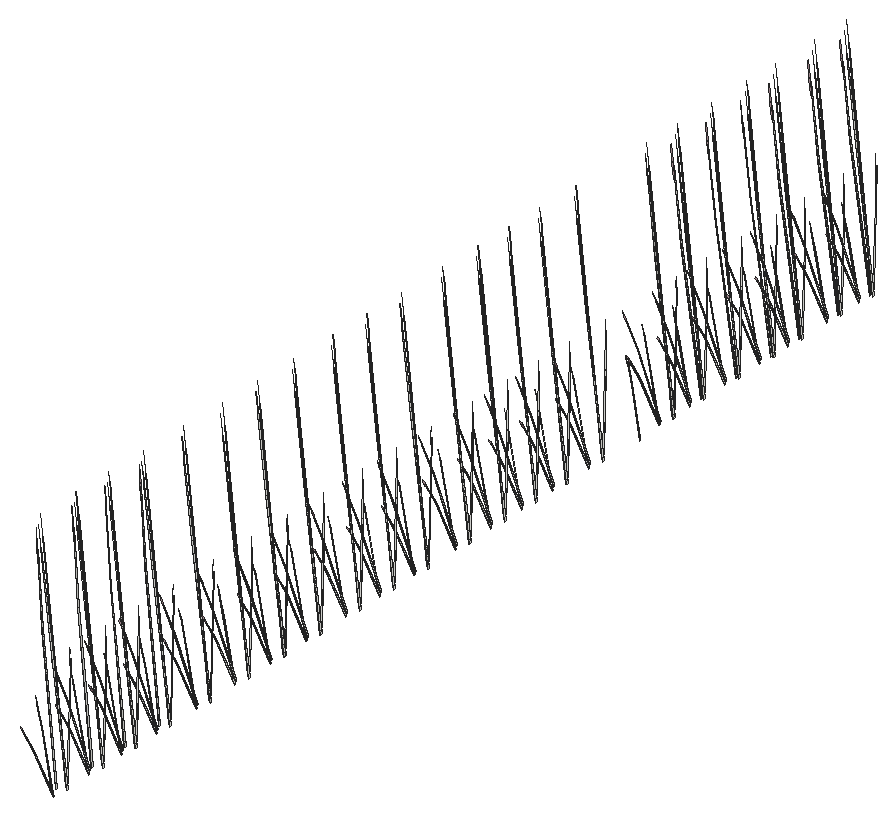
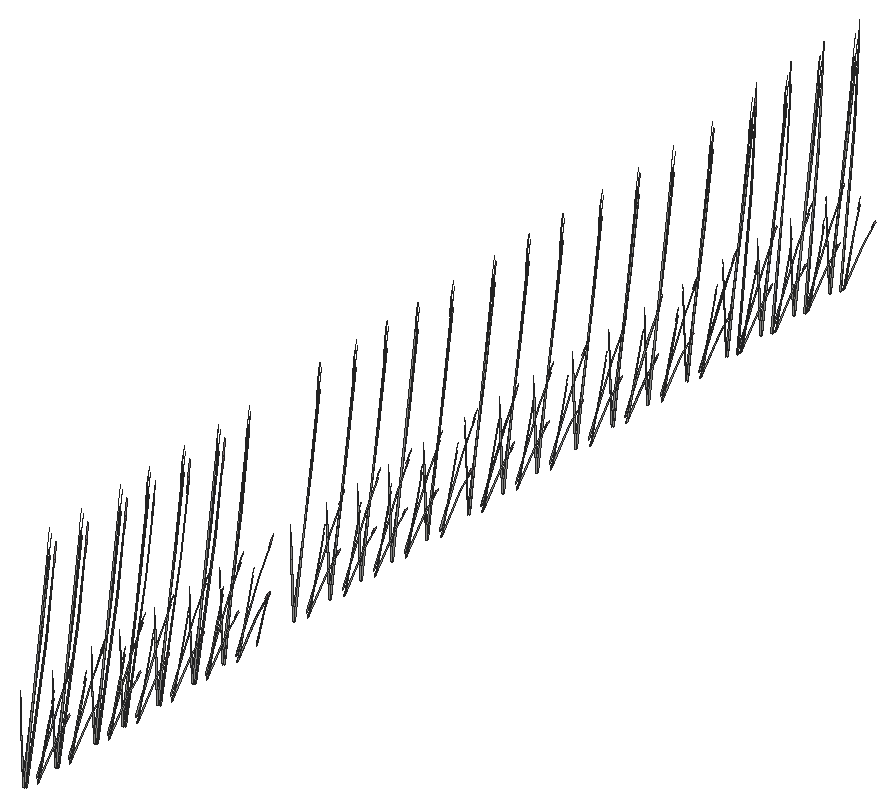
# SketchUp Ruby script. Lengths in inches.
U = 1.inch
M = Sketchup.active_model
def pt(a) = Geom::Point3d.new(a.map { |v| v * U })
def face(e, loops, mat)
  f = e.add_face(loops[0].map { |a| pt(a) })
  loops[1..].each { |l| e.add_face(l.map { |a| pt(a) }).erase! }
  f.material = f.back_material = mat if mat
  f
end
# faces: each face lists its corners as indices into pts; further lists are holes
def faces(e, pts, list, mat = nil) = list.each { |f| face(e, (f[0].is_a?(Array) ? f : [f]).map { |l| l.map { |i| pts[i] } }, mat) }
# xy, xz, yz: faces in a plane at the given z, y or x. An outline is a flat list of corners, or four numbers for a rectangle; further outlines are holes
def ring(l) = l.size == 4 ? [[l[0], l[1]], [l[2], l[1]], [l[2], l[3]], [l[0], l[3]]] : l.each_slice(2).to_a
def flat(e, list, mat, &to3) = list.each { |f| face(e, (f[0].is_a?(Array) ? f : [f]).map { |l| ring(l).map { |u, v| to3.(u, v) } }, mat) }
def xy(e, z, list, mat = nil) = flat(e, list, mat) { |x, y| [x, y, z] }
def xz(e, y, list, mat = nil) = flat(e, list, mat) { |x, z| [x, y, z] }
def yz(e, x, list, mat = nil) = flat(e, list, mat) { |y, z| [x, y, z] }
def lines(e, pts, list) = list.each { |a, b| e.add_line(pt(pts[a]), pt(pts[b])) }
# prism: a flat outline (further loops are holes) pulled along v
def prism(e, loops, v, mat = nil)
  f = face(e, loops, mat); d = Geom::Vector3d.new(v.map { |x| x * U })
  f.pushpull(f.normal.samedirection?(d) ? d.length : -d.length)
end
def box(e, o, s, mat = nil) = prism(e, [[o, [o[0] + s[0], o[1], o[2]], [o[0] + s[0], o[1] + s[1], o[2]], [o[0], o[1] + s[1], o[2]]]], [0, 0, s[2]], mat)
def at(x, y, z, deg = 0) = Geom::Transformation.translation(pt([x, y, z])) * Geom::Transformation.rotation(ORIGIN, Z_AXIS, deg.degrees)
def axes(o, x, y, z) = Geom::Transformation.new([*x, 0, *y, 0, *z, 0, *pt(o).to_a, 1])
def part(name) = M.definitions.add(name)
# library, detail: a bought-in or finely detailed component or shape, given as its bounding box
def library(name, o, s) = part(name).tap { |d| box(d.entities, o, s) }
def detail(e, o, s) = box(e.add_group.entities, o, s)
def put(e, d, t, mat = nil) = e.add_instance(d, t).tap { |i| i.material = mat if mat }
def group(e, t, mat = nil) = e.add_group.tap { |g| g.transformation = t; g.material = mat if mat }.entities
root = M.entities
M.materials.add("LightPink_Translucent").color = [144, 107, 117]
M.materials["LightPink_Translucent"].alpha = 0.75
c1 = part("blade")
p = [[2.15,0.21,22],[0,0.17,0],[0.09,0.45,0],[2.18,0.31,22],[2.29,0.31,22],[0.38,0.45,0],
  [2.48,0.24,33],[2.49,0.24,33],[2.48,0.22,33]]
faces(c1.entities,p,[[0,1,2,3],[4,5,2,3],[6,3,4,7],[8,0,3,6]])
c2 = part("seeds")
p = [[0.3,-0.1,1.38],[-0.01,-0.03,1.59],[-0.01,-0.03,0.03],[0.14,-0.07,-0.07],[0.29,-0.03,3],[0.15,0.01,3.11]]
faces(c2.entities,p,[[0,1,2,3],[1,0,4,5]],"LightPink_Translucent")
c3 = part("blade with seeds")
put(c3.entities,c1,at(0,0,0))
put(c3.entities,c2,axes([2.4,0.25,30.99],[1.5799,-0.05474,1.17369],[-0.12525,1.92788,0.29478],[-0.07173,-0.02425,1.56792]))
put(root,c3,axes([332.39,452.5,49.78],[-0.47255,-0.19538,-0.43871],[0.28245,-0.35034,0],[-0.10763,-0.0445,1.3917]))
put(root,c3,axes([332.39,462.02,49.78],[-0.47255,-0.19538,-0.43871],[0.28245,-0.35034,0],[-0.10763,-0.0445,1.3917]))
put(root,c3,axes([332.39,471.57,49.78],[-0.47255,-0.19538,-0.43871],[0.28245,-0.35034,0],[-0.10763,-0.0445,1.3917]))
put(root,c3,axes([332.39,479.37,49.78],[-0.47255,-0.19538,-0.43871],[0.28245,-0.35034,0],[-0.10763,-0.0445,1.3917]))
put(root,c3,axes([332.39,490.07,49.78],[-0.47255,-0.19538,-0.43871],[0.28245,-0.35034,0],[-0.10763,-0.0445,1.3917]))
put(root,c3,axes([332.39,498.85,49.78],[-0.47255,-0.19538,-0.43871],[0.28245,-0.35034,0],[-0.10763,-0.0445,1.3917]))
put(root,c3,axes([332.18,275.01,49.32],[-0.04891,0.05148,1.55816],[-0.49427,0.11098,-0.23804],[-0.1194,-0.10096,0.26541]))
put(root,c3,axes([332.18,284.8125,49.32],[-0.04891,0.05148,1.55816],[-0.49427,0.11098,-0.23804],[-0.1194,-0.10096,0.26541]))
put(root,c3,axes([332.18,293.79,49.32],[-0.04891,0.05148,1.55816],[-0.49427,0.11098,-0.23804],[-0.1194,-0.10096,0.26541]))
put(root,c3,axes([332.18,303.27,49.32],[-0.04891,0.05148,1.55816],[-0.49427,0.11098,-0.23804],[-0.1194,-0.10096,0.26541]))
put(root,c3,axes([332.18,314.26,49.32],[-0.04891,0.05148,1.55816],[-0.49427,0.11098,-0.23804],[-0.1194,-0.10096,0.26541]))
put(root,c3,axes([332.18,324.86,49.32],[-0.04891,0.05148,1.55816],[-0.49427,0.11098,-0.23804],[-0.1194,-0.10096,0.26541]))
put(root,c3,axes([332.18,334.5625,49.32],[-0.04891,0.05148,1.55816],[-0.49427,0.11098,-0.23804],[-0.1194,-0.10096,0.26541]))
put(root,c3,axes([332.18,344.5,49.32],[-0.04891,0.05148,1.55816],[-0.49427,0.11098,-0.23804],[-0.1194,-0.10096,0.26541]))
put(root,c3,axes([332.18,355.22,49.32],[-0.04891,0.05148,1.55816],[-0.49427,0.11098,-0.23804],[-0.1194,-0.10096,0.26541]))
put(root,c3,axes([332.18,364.55,49.32],[-0.04891,0.05148,1.55816],[-0.49427,0.11098,-0.23804],[-0.1194,-0.10096,0.26541]))
put(root,c3,axes([332.18,374.02,49.32],[-0.04891,0.05148,1.55816],[-0.49427,0.11098,-0.23804],[-0.1194,-0.10096,0.26541]))
put(root,c3,axes([332.18,385.33,49.32],[-0.04891,0.05148,1.55816],[-0.49427,0.11098,-0.23804],[-0.1194,-0.10096,0.26541]))
put(root,c3,axes([332.18,395.01,49.32],[-0.04891,0.05148,1.55816],[-0.49427,0.11098,-0.23804],[-0.1194,-0.10096,0.26541]))
put(root,c3,axes([332.18,403.47,49.32],[-0.04891,0.05148,1.55816],[-0.49427,0.11098,-0.23804],[-0.1194,-0.10096,0.26541]))
put(root,c3,axes([332.18,411.9375,49.32],[-0.04891,0.05148,1.55816],[-0.49427,0.11098,-0.23804],[-0.1194,-0.10096,0.26541]))
put(root,c3,axes([332.18,421.83,49.32],[-0.04891,0.05148,1.55816],[-0.49427,0.11098,-0.23804],[-0.1194,-0.10096,0.26541]))
put(root,c3,axes([332.18,441.22,49.32],[-0.04891,0.05148,1.55816],[-0.49427,0.11098,-0.23804],[-0.1194,-0.10096,0.26541]))
put(root,c3,axes([332.18,449.59,49.32],[-0.04891,0.05148,1.55816],[-0.49427,0.11098,-0.23804],[-0.1194,-0.10096,0.26541]))
put(root,c3,axes([332.18,459.11,49.32],[-0.04891,0.05148,1.55816],[-0.49427,0.11098,-0.23804],[-0.1194,-0.10096,0.26541]))
put(root,c3,axes([332.18,468.66,49.32],[-0.04891,0.05148,1.55816],[-0.49427,0.11098,-0.23804],[-0.1194,-0.10096,0.26541]))
put(root,c3,axes([332.18,476.46,49.32],[-0.04891,0.05148,1.55816],[-0.49427,0.11098,-0.23804],[-0.1194,-0.10096,0.26541]))
put(root,c3,axes([332.18,487.16,49.32],[-0.04891,0.05148,1.55816],[-0.49427,0.11098,-0.23804],[-0.1194,-0.10096,0.26541]))
put(root,c3,axes([332.18,495.9375,49.32],[-0.04891,0.05148,1.55816],[-0.49427,0.11098,-0.23804],[-0.1194,-0.10096,0.26541]))
put(root,c3,axes([332.68,278.16,50.1],[-0.31568,0.39156,0],[-0.52815,-0.21836,-0.456],[-0.12029,-0.04973,1.44655]))
put(root,c3,axes([332.68,287.96,50.1],[-0.31568,0.39156,0],[-0.52815,-0.21836,-0.456],[-0.12029,-0.04973,1.44655]))
put(root,c3,axes([332.68,296.93,50.1],[-0.31568,0.39156,0],[-0.52815,-0.21836,-0.456],[-0.12029,-0.04973,1.44655]))
put(root,c3,axes([332.68,306.42,50.1],[-0.31568,0.39156,0],[-0.52815,-0.21836,-0.456],[-0.12029,-0.04973,1.44655]))
put(root,c3,axes([332.68,317.41,50.1],[-0.31568,0.39156,0],[-0.52815,-0.21836,-0.456],[-0.12029,-0.04973,1.44655]))
put(root,c3,axes([332.68,328.01,50.1],[-0.31568,0.39156,0],[-0.52815,-0.21836,-0.456],[-0.12029,-0.04973,1.44655]))
put(root,c3,axes([332.68,337.71,50.1],[-0.31568,0.39156,0],[-0.52815,-0.21836,-0.456],[-0.12029,-0.04973,1.44655]))
put(root,c3,axes([332.68,347.65,50.1],[-0.31568,0.39156,0],[-0.52815,-0.21836,-0.456],[-0.12029,-0.04973,1.44655]))
put(root,c3,axes([332.68,358.37,50.1],[-0.31568,0.39156,0],[-0.52815,-0.21836,-0.456],[-0.12029,-0.04973,1.44655]))
put(root,c3,axes([332.68,367.69,50.1],[-0.31568,0.39156,0],[-0.52815,-0.21836,-0.456],[-0.12029,-0.04973,1.44655]))
put(root,c3,axes([332.68,377.17,50.1],[-0.31568,0.39156,0],[-0.52815,-0.21836,-0.456],[-0.12029,-0.04973,1.44655]))
put(root,c3,axes([332.68,388.47,50.1],[-0.31568,0.39156,0],[-0.52815,-0.21836,-0.456],[-0.12029,-0.04973,1.44655]))
put(root,c3,axes([332.68,398.16,50.1],[-0.31568,0.39156,0],[-0.52815,-0.21836,-0.456],[-0.12029,-0.04973,1.44655]))
put(root,c3,axes([332.68,406.62,50.1],[-0.31568,0.39156,0],[-0.52815,-0.21836,-0.456],[-0.12029,-0.04973,1.44655]))
put(root,c3,axes([332.68,415.08,50.1],[-0.31568,0.39156,0],[-0.52815,-0.21836,-0.456],[-0.12029,-0.04973,1.44655]))
put(root,c3,axes([332.68,424.98,50.1],[-0.31568,0.39156,0],[-0.52815,-0.21836,-0.456],[-0.12029,-0.04973,1.44655]))
put(root,c3,axes([332.68,444.37,50.1],[-0.31568,0.39156,0],[-0.52815,-0.21836,-0.456],[-0.12029,-0.04973,1.44655]))
put(root,c3,axes([332.68,452.74,50.1],[-0.31568,0.39156,0],[-0.52815,-0.21836,-0.456],[-0.12029,-0.04973,1.44655]))
put(root,c3,axes([332.68,462.25,50.1],[-0.31568,0.39156,0],[-0.52815,-0.21836,-0.456],[-0.12029,-0.04973,1.44655]))
put(root,c3,axes([332.68,471.81,50.1],[-0.31568,0.39156,0],[-0.52815,-0.21836,-0.456],[-0.12029,-0.04973,1.44655]))
put(root,c3,axes([332.68,479.61,50.1],[-0.31568,0.39156,0],[-0.52815,-0.21836,-0.456],[-0.12029,-0.04973,1.44655]))
put(root,c3,axes([332.68,490.31,50.1],[-0.31568,0.39156,0],[-0.52815,-0.21836,-0.456],[-0.12029,-0.04973,1.44655]))
put(root,c3,axes([332.68,499.08,50.1],[-0.31568,0.39156,0],[-0.52815,-0.21836,-0.456],[-0.12029,-0.04973,1.44655]))
put(root,c3,axes([332.84,434.68,49.32],[0.06773,0.03904,1.55816],[0.11484,0.36171,-0.23804],[-0.15011,0.07713,0.26541]))
put(root,c3,axes([332.1,278.72,50.29],[0.15933,-0.06164,1.26356],[0.39339,0.18587,-0.27174],[-0.11709,0.16083,0.54024]))
put(root,c3,axes([332.1,288.52,50.29],[0.15933,-0.06164,1.26356],[0.39339,0.18587,-0.27174],[-0.11709,0.16083,0.54024]))
put(root,c3,axes([332.1,297.5,50.29],[0.15933,-0.06164,1.26356],[0.39339,0.18587,-0.27174],[-0.11709,0.16083,0.54024]))
put(root,c3,axes([332.1,306.99,50.29],[0.15933,-0.06164,1.26356],[0.39339,0.18587,-0.27174],[-0.11709,0.16083,0.54024]))
put(root,c3,axes([332.1,317.97,50.29],[0.15933,-0.06164,1.26356],[0.39339,0.18587,-0.27174],[-0.11709,0.16083,0.54024]))
put(root,c3,axes([332.1,328.57,50.29],[0.15933,-0.06164,1.26356],[0.39339,0.18587,-0.27174],[-0.11709,0.16083,0.54024]))
put(root,c3,axes([332.1,338.28,50.29],[0.15933,-0.06164,1.26356],[0.39339,0.18587,-0.27174],[-0.11709,0.16083,0.54024]))
put(root,c3,axes([332.1,348.21,50.29],[0.15933,-0.06164,1.26356],[0.39339,0.18587,-0.27174],[-0.11709,0.16083,0.54024]))
put(root,c3,axes([332.1,358.93,50.29],[0.15933,-0.06164,1.26356],[0.39339,0.18587,-0.27174],[-0.11709,0.16083,0.54024]))
put(root,c3,axes([332.1,368.26,50.29],[0.15933,-0.06164,1.26356],[0.39339,0.18587,-0.27174],[-0.11709,0.16083,0.54024]))
put(root,c3,axes([332.1,377.73,50.29],[0.15933,-0.06164,1.26356],[0.39339,0.18587,-0.27174],[-0.11709,0.16083,0.54024]))
put(root,c3,axes([332.1,389.04,50.29],[0.15933,-0.06164,1.26356],[0.39339,0.18587,-0.27174],[-0.11709,0.16083,0.54024]))
put(root,c3,axes([332.1,398.72,50.29],[0.15933,-0.06164,1.26356],[0.39339,0.18587,-0.27174],[-0.11709,0.16083,0.54024]))
put(root,c3,axes([332.1,407.18,50.29],[0.15933,-0.06164,1.26356],[0.39339,0.18587,-0.27174],[-0.11709,0.16083,0.54024]))
put(root,c3,axes([332.1,415.65,50.29],[0.15933,-0.06164,1.26356],[0.39339,0.18587,-0.27174],[-0.11709,0.16083,0.54024]))
put(root,c3,axes([332.1,425.55,50.29],[0.15933,-0.06164,1.26356],[0.39339,0.18587,-0.27174],[-0.11709,0.16083,0.54024]))
put(root,c3,axes([332.1,444.93,50.29],[0.15933,-0.06164,1.26356],[0.39339,0.18587,-0.27174],[-0.11709,0.16083,0.54024]))
put(root,c3,axes([332.1,453.31,50.29],[0.15933,-0.06164,1.26356],[0.39339,0.18587,-0.27174],[-0.11709,0.16083,0.54024]))
put(root,c3,axes([332.1,462.82,50.29],[0.15933,-0.06164,1.26356],[0.39339,0.18587,-0.27174],[-0.11709,0.16083,0.54024]))
put(root,c3,axes([332.1,472.375,50.29],[0.15933,-0.06164,1.26356],[0.39339,0.18587,-0.27174],[-0.11709,0.16083,0.54024]))
put(root,c3,axes([332.1,480.17,50.29],[0.15933,-0.06164,1.26356],[0.39339,0.18587,-0.27174],[-0.11709,0.16083,0.54024]))
put(root,c3,axes([332.1,490.87,50.29],[0.15933,-0.06164,1.26356],[0.39339,0.18587,-0.27174],[-0.11709,0.16083,0.54024]))
put(root,c3,axes([332.1,499.65,50.29],[0.15933,-0.06164,1.26356],[0.39339,0.18587,-0.27174],[-0.11709,0.16083,0.54024]))
put(root,c3,axes([331.88,275.21,49.88],[-0.14565,0.31907,-0.0344],[-0.44829,-0.09815,-0.15595],[-0.06806,-0.05219,0.51438]))
put(root,c3,axes([331.88,285.01,49.88],[-0.14565,0.31907,-0.0344],[-0.44829,-0.09815,-0.15595],[-0.06806,-0.05219,0.51438]))
put(root,c3,axes([331.88,293.99,49.88],[-0.14565,0.31907,-0.0344],[-0.44829,-0.09815,-0.15595],[-0.06806,-0.05219,0.51438]))
put(root,c3,axes([331.88,303.47,49.88],[-0.14565,0.31907,-0.0344],[-0.44829,-0.09815,-0.15595],[-0.06806,-0.05219,0.51438]))
put(root,c3,axes([331.88,314.46,49.88],[-0.14565,0.31907,-0.0344],[-0.44829,-0.09815,-0.15595],[-0.06806,-0.05219,0.51438]))
put(root,c3,axes([331.88,325.06,49.88],[-0.14565,0.31907,-0.0344],[-0.44829,-0.09815,-0.15595],[-0.06806,-0.05219,0.51438]))
put(root,c3,axes([331.88,334.76,49.88],[-0.14565,0.31907,-0.0344],[-0.44829,-0.09815,-0.15595],[-0.06806,-0.05219,0.51438]))
put(root,c3,axes([331.88,344.7,49.88],[-0.14565,0.31907,-0.0344],[-0.44829,-0.09815,-0.15595],[-0.06806,-0.05219,0.51438]))
put(root,c3,axes([331.88,355.42,49.88],[-0.14565,0.31907,-0.0344],[-0.44829,-0.09815,-0.15595],[-0.06806,-0.05219,0.51438]))
put(root,c3,axes([331.88,364.75,49.88],[-0.14565,0.31907,-0.0344],[-0.44829,-0.09815,-0.15595],[-0.06806,-0.05219,0.51438]))
put(root,c3,axes([331.88,374.22,49.88],[-0.14565,0.31907,-0.0344],[-0.44829,-0.09815,-0.15595],[-0.06806,-0.05219,0.51438]))
put(root,c3,axes([331.88,385.53,49.88],[-0.14565,0.31907,-0.0344],[-0.44829,-0.09815,-0.15595],[-0.06806,-0.05219,0.51438]))
put(root,c3,axes([331.88,395.21,49.88],[-0.14565,0.31907,-0.0344],[-0.44829,-0.09815,-0.15595],[-0.06806,-0.05219,0.51438]))
put(root,c3,axes([331.88,403.67,49.88],[-0.14565,0.31907,-0.0344],[-0.44829,-0.09815,-0.15595],[-0.06806,-0.05219,0.51438]))
put(root,c3,axes([331.88,412.14,49.88],[-0.14565,0.31907,-0.0344],[-0.44829,-0.09815,-0.15595],[-0.06806,-0.05219,0.51438]))
put(root,c3,axes([331.88,422.03,49.88],[-0.14565,0.31907,-0.0344],[-0.44829,-0.09815,-0.15595],[-0.06806,-0.05219,0.51438]))
put(root,c3,axes([331.88,441.42,49.88],[-0.14565,0.31907,-0.0344],[-0.44829,-0.09815,-0.15595],[-0.06806,-0.05219,0.51438]))
put(root,c3,axes([331.88,449.79,49.88],[-0.14565,0.31907,-0.0344],[-0.44829,-0.09815,-0.15595],[-0.06806,-0.05219,0.51438]))
put(root,c3,axes([331.88,459.31,49.88],[-0.14565,0.31907,-0.0344],[-0.44829,-0.09815,-0.15595],[-0.06806,-0.05219,0.51438]))
put(root,c3,axes([331.88,468.86,49.88],[-0.14565,0.31907,-0.0344],[-0.44829,-0.09815,-0.15595],[-0.06806,-0.05219,0.51438]))
put(root,c3,axes([331.88,476.66,49.88],[-0.14565,0.31907,-0.0344],[-0.44829,-0.09815,-0.15595],[-0.06806,-0.05219,0.51438]))
put(root,c3,axes([331.88,487.36,49.88],[-0.14565,0.31907,-0.0344],[-0.44829,-0.09815,-0.15595],[-0.06806,-0.05219,0.51438]))
put(root,c3,axes([331.88,496.14,49.88],[-0.14565,0.31907,-0.0344],[-0.44829,-0.09815,-0.15595],[-0.06806,-0.05219,0.51438]))
put(root,c3,axes([332.55,284.61,50.29],[-0.03058,0.12783,1.26356],[-0.44698,0.10701,-0.27174],[-0.10448,-0.16522,0.54024]))
put(root,c3,axes([332.55,293.58,50.29],[-0.03058,0.12783,1.26356],[-0.44698,0.10701,-0.27174],[-0.10448,-0.16522,0.54024]))
put(root,c3,axes([332.55,303.07,50.29],[-0.03058,0.12783,1.26356],[-0.44698,0.10701,-0.27174],[-0.10448,-0.16522,0.54024]))
put(root,c3,axes([332.55,314.06,50.29],[-0.03058,0.12783,1.26356],[-0.44698,0.10701,-0.27174],[-0.10448,-0.16522,0.54024]))
put(root,c3,axes([332.55,324.66,50.29],[-0.03058,0.12783,1.26356],[-0.44698,0.10701,-0.27174],[-0.10448,-0.16522,0.54024]))
put(root,c3,axes([332.55,334.36,50.29],[-0.03058,0.12783,1.26356],[-0.44698,0.10701,-0.27174],[-0.10448,-0.16522,0.54024]))
put(root,c3,axes([332.55,344.3,50.29],[-0.03058,0.12783,1.26356],[-0.44698,0.10701,-0.27174],[-0.10448,-0.16522,0.54024]))
put(root,c3,axes([332.55,355.02,50.29],[-0.03058,0.12783,1.26356],[-0.44698,0.10701,-0.27174],[-0.10448,-0.16522,0.54024]))
put(root,c3,axes([332.55,364.34,50.29],[-0.03058,0.12783,1.26356],[-0.44698,0.10701,-0.27174],[-0.10448,-0.16522,0.54024]))
put(root,c3,axes([332.55,373.82,50.29],[-0.03058,0.12783,1.26356],[-0.44698,0.10701,-0.27174],[-0.10448,-0.16522,0.54024]))
put(root,c3,axes([332.55,385.125,50.29],[-0.03058,0.12783,1.26356],[-0.44698,0.10701,-0.27174],[-0.10448,-0.16522,0.54024]))
put(root,c3,axes([332.55,394.81,50.29],[-0.03058,0.12783,1.26356],[-0.44698,0.10701,-0.27174],[-0.10448,-0.16522,0.54024]))
put(root,c3,axes([332.55,403.27,50.29],[-0.03058,0.12783,1.26356],[-0.44698,0.10701,-0.27174],[-0.10448,-0.16522,0.54024]))
put(root,c3,axes([332.55,411.73,50.29],[-0.03058,0.12783,1.26356],[-0.44698,0.10701,-0.27174],[-0.10448,-0.16522,0.54024]))
put(root,c3,axes([332.55,421.63,50.29],[-0.03058,0.12783,1.26356],[-0.44698,0.10701,-0.27174],[-0.10448,-0.16522,0.54024]))
put(root,c3,axes([332.55,441.02,50.29],[-0.03058,0.12783,1.26356],[-0.44698,0.10701,-0.27174],[-0.10448,-0.16522,0.54024]))
put(root,c3,axes([332.55,449.39,50.29],[-0.03058,0.12783,1.26356],[-0.44698,0.10701,-0.27174],[-0.10448,-0.16522,0.54024]))
put(root,c3,axes([332.55,458.9,50.29],[-0.03058,0.12783,1.26356],[-0.44698,0.10701,-0.27174],[-0.10448,-0.16522,0.54024]))
put(root,c3,axes([332.55,468.46,50.29],[-0.03058,0.12783,1.26356],[-0.44698,0.10701,-0.27174],[-0.10448,-0.16522,0.54024]))
put(root,c3,axes([332.55,476.26,50.29],[-0.03058,0.12783,1.26356],[-0.44698,0.10701,-0.27174],[-0.10448,-0.16522,0.54024]))
put(root,c3,axes([332.55,486.96,50.29],[-0.03058,0.12783,1.26356],[-0.44698,0.10701,-0.27174],[-0.10448,-0.16522,0.54024]))
put(root,c3,axes([332.55,495.73,50.29],[-0.03058,0.12783,1.26356],[-0.44698,0.10701,-0.27174],[-0.10448,-0.16522,0.54024]))
put(root,c3,axes([333.68,277.23,50.36],[-0.50979,0.25942,-0.25709],[-0.339,-0.36656,-0.44182],[-0.12578,-0.03723,1.41118]))
put(root,c3,axes([333.68,287.03,50.36],[-0.50979,0.25942,-0.25709],[-0.339,-0.36656,-0.44182],[-0.12578,-0.03723,1.41118]))
put(root,c3,axes([333.68,296.01,50.36],[-0.50979,0.25942,-0.25709],[-0.339,-0.36656,-0.44182],[-0.12578,-0.03723,1.41118]))
put(root,c3,axes([333.68,305.49,50.36],[-0.50979,0.25942,-0.25709],[-0.339,-0.36656,-0.44182],[-0.12578,-0.03723,1.41118]))
put(root,c3,axes([333.68,316.48,50.36],[-0.50979,0.25942,-0.25709],[-0.339,-0.36656,-0.44182],[-0.12578,-0.03723,1.41118]))
put(root,c3,axes([333.68,327.08,50.36],[-0.50979,0.25942,-0.25709],[-0.339,-0.36656,-0.44182],[-0.12578,-0.03723,1.41118]))
put(root,c3,axes([333.68,336.78,50.36],[-0.50979,0.25942,-0.25709],[-0.339,-0.36656,-0.44182],[-0.12578,-0.03723,1.41118]))
put(root,c3,axes([333.68,346.72,50.36],[-0.50979,0.25942,-0.25709],[-0.339,-0.36656,-0.44182],[-0.12578,-0.03723,1.41118]))
put(root,c3,axes([333.68,357.44,50.36],[-0.50979,0.25942,-0.25709],[-0.339,-0.36656,-0.44182],[-0.12578,-0.03723,1.41118]))
put(root,c3,axes([333.68,366.77,50.36],[-0.50979,0.25942,-0.25709],[-0.339,-0.36656,-0.44182],[-0.12578,-0.03723,1.41118]))
put(root,c3,axes([333.68,376.24,50.36],[-0.50979,0.25942,-0.25709],[-0.339,-0.36656,-0.44182],[-0.12578,-0.03723,1.41118]))
put(root,c3,axes([333.68,387.55,50.36],[-0.50979,0.25942,-0.25709],[-0.339,-0.36656,-0.44182],[-0.12578,-0.03723,1.41118]))
put(root,c3,axes([333.68,397.23,50.36],[-0.50979,0.25942,-0.25709],[-0.339,-0.36656,-0.44182],[-0.12578,-0.03723,1.41118]))
put(root,c3,axes([333.68,405.69,50.36],[-0.50979,0.25942,-0.25709],[-0.339,-0.36656,-0.44182],[-0.12578,-0.03723,1.41118]))
put(root,c3,axes([333.68,414.16,50.36],[-0.50979,0.25942,-0.25709],[-0.339,-0.36656,-0.44182],[-0.12578,-0.03723,1.41118]))
put(root,c3,axes([333.68,424.06,50.36],[-0.50979,0.25942,-0.25709],[-0.339,-0.36656,-0.44182],[-0.12578,-0.03723,1.41118]))
put(root,c3,axes([333.68,443.44,50.36],[-0.50979,0.25942,-0.25709],[-0.339,-0.36656,-0.44182],[-0.12578,-0.03723,1.41118]))
put(root,c3,axes([333.68,451.8125,50.36],[-0.50979,0.25942,-0.25709],[-0.339,-0.36656,-0.44182],[-0.12578,-0.03723,1.41118]))
put(root,c3,axes([333.68,461.33,50.36],[-0.50979,0.25942,-0.25709],[-0.339,-0.36656,-0.44182],[-0.12578,-0.03723,1.41118]))
put(root,c3,axes([333.68,470.88,50.36],[-0.50979,0.25942,-0.25709],[-0.339,-0.36656,-0.44182],[-0.12578,-0.03723,1.41118]))
put(root,c3,axes([333.68,478.68,50.36],[-0.50979,0.25942,-0.25709],[-0.339,-0.36656,-0.44182],[-0.12578,-0.03723,1.41118]))
put(root,c3,axes([333.68,489.38,50.36],[-0.50979,0.25942,-0.25709],[-0.339,-0.36656,-0.44182],[-0.12578,-0.03723,1.41118]))
put(root,c3,axes([333.68,498.16,50.36],[-0.50979,0.25942,-0.25709],[-0.339,-0.36656,-0.44182],[-0.12578,-0.03723,1.41118]))
put(root,c3,axes([331.64,276.66,50.1],[-0.63136,0,0],[0,-0.43672,-0.456],[0,-0.09947,1.44655]))
put(root,c3,axes([331.64,286.47,50.1],[-0.63136,0,0],[0,-0.43672,-0.456],[0,-0.09947,1.44655]))
put(root,c3,axes([331.64,295.44,50.1],[-0.63136,0,0],[0,-0.43672,-0.456],[0,-0.09947,1.44655]))
put(root,c3,axes([331.64,304.93,50.1],[-0.63136,0,0],[0,-0.43672,-0.456],[0,-0.09947,1.44655]))
